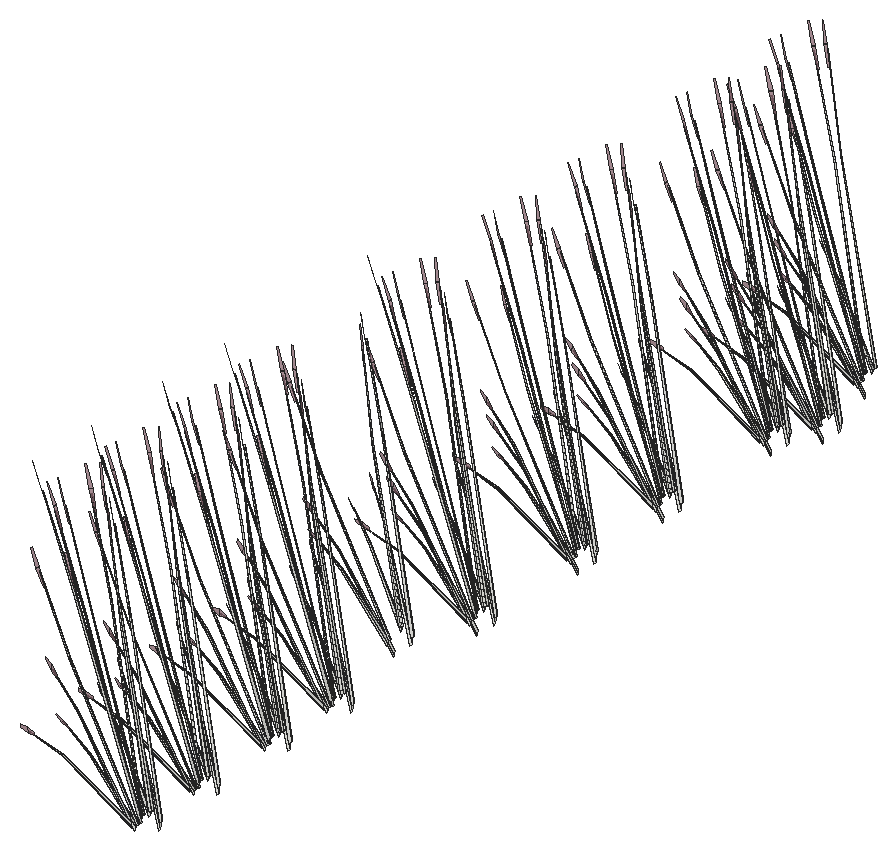
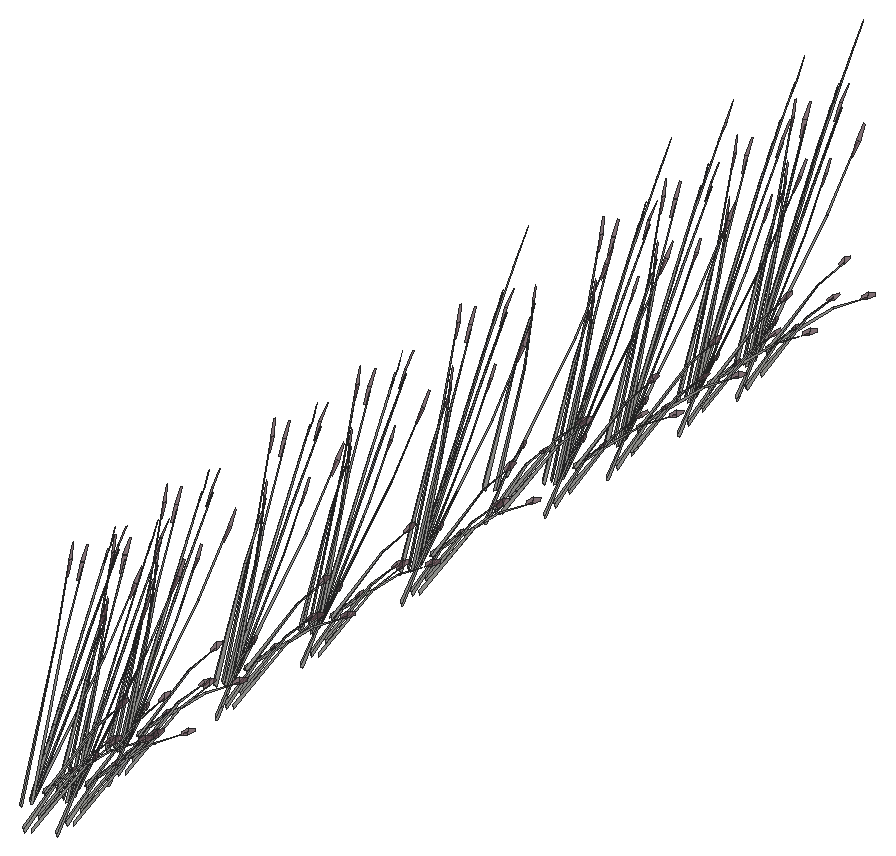
# SketchUp Ruby script. Lengths in inches.
U = 1.inch
M = Sketchup.active_model
def pt(a) = Geom::Point3d.new(a.map { |v| v * U })
def face(e, loops, mat)
  f = e.add_face(loops[0].map { |a| pt(a) })
  loops[1..].each { |l| e.add_face(l.map { |a| pt(a) }).erase! }
  f.material = f.back_material = mat if mat
  f
end
# faces: each face lists its corners as indices into pts; further lists are holes
def faces(e, pts, list, mat = nil) = list.each { |f| face(e, (f[0].is_a?(Array) ? f : [f]).map { |l| l.map { |i| pts[i] } }, mat) }
# xy, xz, yz: faces in a plane at the given z, y or x. An outline is a flat list of corners, or four numbers for a rectangle; further outlines are holes
def ring(l) = l.size == 4 ? [[l[0], l[1]], [l[2], l[1]], [l[2], l[3]], [l[0], l[3]]] : l.each_slice(2).to_a
def flat(e, list, mat, &to3) = list.each { |f| face(e, (f[0].is_a?(Array) ? f : [f]).map { |l| ring(l).map { |u, v| to3.(u, v) } }, mat) }
def xy(e, z, list, mat = nil) = flat(e, list, mat) { |x, y| [x, y, z] }
def xz(e, y, list, mat = nil) = flat(e, list, mat) { |x, z| [x, y, z] }
def yz(e, x, list, mat = nil) = flat(e, list, mat) { |y, z| [x, y, z] }
def lines(e, pts, list) = list.each { |a, b| e.add_line(pt(pts[a]), pt(pts[b])) }
# prism: a flat outline (further loops are holes) pulled along v
def prism(e, loops, v, mat = nil)
  f = face(e, loops, mat); d = Geom::Vector3d.new(v.map { |x| x * U })
  f.pushpull(f.normal.samedirection?(d) ? d.length : -d.length)
end
def box(e, o, s, mat = nil) = prism(e, [[o, [o[0] + s[0], o[1], o[2]], [o[0] + s[0], o[1] + s[1], o[2]], [o[0], o[1] + s[1], o[2]]]], [0, 0, s[2]], mat)
def at(x, y, z, deg = 0) = Geom::Transformation.translation(pt([x, y, z])) * Geom::Transformation.rotation(ORIGIN, Z_AXIS, deg.degrees)
def axes(o, x, y, z) = Geom::Transformation.new([*x, 0, *y, 0, *z, 0, *pt(o).to_a, 1])
def part(name) = M.definitions.add(name)
# library, detail: a bought-in or finely detailed component or shape, given as its bounding box
def library(name, o, s) = part(name).tap { |d| box(d.entities, o, s) }
def detail(e, o, s) = box(e.add_group.entities, o, s)
def put(e, d, t, mat = nil) = e.add_instance(d, t).tap { |i| i.material = mat if mat }
def group(e, t, mat = nil) = e.add_group.tap { |g| g.transformation = t; g.material = mat if mat }.entities
root = M.entities
M.materials.add("LightPink_Translucent").color = [144, 107, 117]
M.materials["LightPink_Translucent"].alpha = 0.75
c1 = part("blade")
p = [[2.15,0.21,22],[0,0.17,0],[0.09,0.45,0],[2.18,0.31,22],[2.29,0.31,22],[0.38,0.45,0],
  [2.48,0.24,33],[2.49,0.24,33],[2.48,0.22,33]]
faces(c1.entities,p,[[0,1,2,3],[4,5,2,3],[6,3,4,7],[8,0,3,6]])
c2 = part("seeds")
p = [[0.3,-0.1,1.38],[-0.01,-0.03,1.59],[-0.01,-0.03,0.03],[0.14,-0.07,-0.07],[0.29,-0.03,3],[0.15,0.01,3.11]]
faces(c2.entities,p,[[0,1,2,3],[1,0,4,5]],"LightPink_Translucent")
c3 = part("blade with seeds")
put(c3.entities,c1,at(0,0,0))
put(c3.entities,c2,axes([2.4,0.25,30.99],[1.5799,-0.05474,1.17369],[-0.12525,1.92788,0.29478],[-0.07173,-0.02425,1.56792]))
put(root,c3,axes([340.12,103.96,7.49],[0.02269,0.10283,1.76342],[-0.45738,0.53699,-0.26939],[-0.32488,-0.02707,0.30037]))
put(root,c3,axes([340.12,117.96,3.79],[0.02269,0.10283,1.76342],[-0.45738,0.53699,-0.26939],[-0.32488,-0.02707,0.30037]))
put(root,c3,axes([340.12,134.9,3.79],[0.02269,0.10283,1.76342],[-0.45738,0.53699,-0.26939],[-0.32488,-0.02707,0.30037]))
put(root,c3,axes([340.12,149.25,3.79],[0.02269,0.10283,1.76342],[-0.45738,0.53699,-0.26939],[-0.32488,-0.02707,0.30037]))
put(root,c3,axes([340.12,167.42,3.79],[0.02269,0.10283,1.76342],[-0.45738,0.53699,-0.26939],[-0.32488,-0.02707,0.30037]))
put(root,c3,axes([340.12,176.07,1.49],[0.02269,0.10283,1.76342],[-0.45738,0.53699,-0.26939],[-0.32488,-0.02707,0.30037]))
put(root,c3,axes([340.12,183.24,3.79],[0.02269,0.10283,1.76342],[-0.45738,0.53699,-0.26939],[-0.32488,-0.02707,0.30037]))
put(root,c3,axes([340.25,59.13,7],[0.06632,0.06511,1.77383],[-0.31973,0.58531,-0.16761],[-0.32381,0.00424,0.31391]))
put(root,c3,axes([340.25,68.96,7],[0.06632,0.06511,1.77383],[-0.31973,0.58531,-0.16761],[-0.32381,0.00424,0.31391]))
put(root,c3,axes([340.25,80.96,7],[0.06632,0.06511,1.77383],[-0.31973,0.58531,-0.16761],[-0.32381,0.00424,0.31391]))
put(root,c3,axes([340.25,91.43,7],[0.06632,0.06511,1.77383],[-0.31973,0.58531,-0.16761],[-0.32381,0.00424,0.31391]))
put(root,c3,axes([340.25,115.51,7],[0.06632,0.06511,1.77383],[-0.31973,0.58531,-0.16761],[-0.32381,0.00424,0.31391]))
put(root,c3,axes([340.25,132.45,7],[0.06632,0.06511,1.77383],[-0.31973,0.58531,-0.16761],[-0.32381,0.00424,0.31391]))
put(root,c3,axes([340.25,146.79,7],[0.06632,0.06511,1.77383],[-0.31973,0.58531,-0.16761],[-0.32381,0.00424,0.31391]))
put(root,c3,axes([340.25,164.96,7],[0.06632,0.06511,1.77383],[-0.31973,0.58531,-0.16761],[-0.32381,0.00424,0.31391]))
put(root,c3,axes([340.25,173.61,4.71],[0.06632,0.06511,1.77383],[-0.31973,0.58531,-0.16761],[-0.32381,0.00424,0.31391]))
put(root,c3,axes([340.25,180.78,7],[0.06632,0.06511,1.77383],[-0.31973,0.58531,-0.16761],[-0.32381,0.00424,0.31391]))
put(root,c3,axes([338.89,64.17,5.06],[0.37283,-0.29571,1.1486],[0.14711,0.46813,0.84392],[-0.26943,0.08382,0.25299]))
put(root,c3,axes([338.89,73.99,5.06],[0.37283,-0.29571,1.1486],[0.14711,0.46813,0.84392],[-0.26943,0.08382,0.25299]))
put(root,c3,axes([338.89,85.99,5.06],[0.37283,-0.29571,1.1486],[0.14711,0.46813,0.84392],[-0.26943,0.08382,0.25299]))
put(root,c3,axes([338.89,96.46,5.06],[0.37283,-0.29571,1.1486],[0.14711,0.46813,0.84392],[-0.26943,0.08382,0.25299]))
put(root,c3,axes([338.89,106.53,8.77],[0.37283,-0.29571,1.1486],[0.14711,0.46813,0.84392],[-0.26943,0.08382,0.25299]))
put(root,c3,axes([338.89,120.54,5.06],[0.37283,-0.29571,1.1486],[0.14711,0.46813,0.84392],[-0.26943,0.08382,0.25299]))
put(root,c3,axes([338.89,137.48,5.06],[0.37283,-0.29571,1.1486],[0.14711,0.46813,0.84392],[-0.26943,0.08382,0.25299]))
put(root,c3,axes([338.89,151.83,5.06],[0.37283,-0.29571,1.1486],[0.14711,0.46813,0.84392],[-0.26943,0.08382,0.25299]))
put(root,c3,axes([338.89,169.99,5.06],[0.37283,-0.29571,1.1486],[0.14711,0.46813,0.84392],[-0.26943,0.08382,0.25299]))
put(root,c3,axes([338.89,178.64,2.77],[0.37283,-0.29571,1.1486],[0.14711,0.46813,0.84392],[-0.26943,0.08382,0.25299]))
put(root,c3,axes([338.89,185.8125,5.06],[0.37283,-0.29571,1.1486],[0.14711,0.46813,0.84392],[-0.26943,0.08382,0.25299]))
put(root,c3,axes([340.99,58.74,7.01],[-0.19249,-0.00461,1.74944],[-0.61281,0.46055,-0.27667],[-0.32697,-0.0941,0.14031]))
put(root,c3,axes([340.99,68.57,7.01],[-0.19249,-0.00461,1.74944],[-0.61281,0.46055,-0.27667],[-0.32697,-0.0941,0.14031]))
put(root,c3,axes([340.99,80.57,7.01],[-0.19249,-0.00461,1.74944],[-0.61281,0.46055,-0.27667],[-0.32697,-0.0941,0.14031]))
put(root,c3,axes([340.99,91.04,7.01],[-0.19249,-0.00461,1.74944],[-0.61281,0.46055,-0.27667],[-0.32697,-0.0941,0.14031]))
put(root,c3,axes([340.99,115.12,7.01],[-0.19249,-0.00461,1.74944],[-0.61281,0.46055,-0.27667],[-0.32697,-0.0941,0.14031]))
put(root,c3,axes([340.99,132.06,7.01],[-0.19249,-0.00461,1.74944],[-0.61281,0.46055,-0.27667],[-0.32697,-0.0941,0.14031]))
put(root,c3,axes([340.99,146.4,7.01],[-0.19249,-0.00461,1.74944],[-0.61281,0.46055,-0.27667],[-0.32697,-0.0941,0.14031]))
put(root,c3,axes([340.99,164.57,7.01],[-0.19249,-0.00461,1.74944],[-0.61281,0.46055,-0.27667],[-0.32697,-0.0941,0.14031]))
put(root,c3,axes([340.99,173.22,4.72],[-0.19249,-0.00461,1.74944],[-0.61281,0.46055,-0.27667],[-0.32697,-0.0941,0.14031]))
put(root,c3,axes([340.99,180.39,7.01],[-0.19249,-0.00461,1.74944],[-0.61281,0.46055,-0.27667],[-0.32697,-0.0941,0.14031]))
put(root,c3,axes([340.2,61.29,7.03],[0.25275,-0.59491,0.48003],[0.83094,0.20343,0.3958],[-0.32677,0.03575,0.9933]))
put(root,c3,axes([340.2,71.12,7.03],[0.25275,-0.59491,0.48003],[0.83094,0.20343,0.3958],[-0.32677,0.03575,0.9933]))
put(root,c3,axes([340.2,83.12,7.03],[0.25275,-0.59491,0.48003],[0.83094,0.20343,0.3958],[-0.32677,0.03575,0.9933]))
put(root,c3,axes([340.2,93.59,7.03],[0.25275,-0.59491,0.48003],[0.83094,0.20343,0.3958],[-0.32677,0.03575,0.9933]))
put(root,c3,axes([340.2,117.66,7.03],[0.25275,-0.59491,0.48003],[0.83094,0.20343,0.3958],[-0.32677,0.03575,0.9933]))
put(root,c3,axes([340.2,134.6,7.03],[0.25275,-0.59491,0.48003],[0.83094,0.20343,0.3958],[-0.32677,0.03575,0.9933]))
put(root,c3,axes([340.2,148.95,7.03],[0.25275,-0.59491,0.48003],[0.83094,0.20343,0.3958],[-0.32677,0.03575,0.9933]))
put(root,c3,axes([340.2,167.12,7.03],[0.25275,-0.59491,0.48003],[0.83094,0.20343,0.3958],[-0.32677,0.03575,0.9933]))
put(root,c3,axes([340.2,175.77,4.73],[0.25275,-0.59491,0.48003],[0.83094,0.20343,0.3958],[-0.32677,0.03575,0.9933]))
put(root,c3,axes([340.2,182.9375,7.03],[0.25275,-0.59491,0.48003],[0.83094,0.20343,0.3958],[-0.32677,0.03575,0.9933]))
put(root,c3,axes([340.5,61.12,7.33],[0.45012,0.59081,-0.1216],[-0.79888,0.29033,-0.67495],[-0.33665,0.07795,1.02557]))
put(root,c3,axes([340.5,70.95,7.33],[0.45012,0.59081,-0.1216],[-0.79888,0.29033,-0.67495],[-0.33665,0.07795,1.02557]))
put(root,c3,axes([340.5,82.95,7.33],[0.45012,0.59081,-0.1216],[-0.79888,0.29033,-0.67495],[-0.33665,0.07795,1.02557]))
put(root,c3,axes([340.5,93.42,7.33],[0.45012,0.59081,-0.1216],[-0.79888,0.29033,-0.67495],[-0.33665,0.07795,1.02557]))
put(root,c3,axes([340.5,117.49,7.33],[0.45012,0.59081,-0.1216],[-0.79888,0.29033,-0.67495],[-0.33665,0.07795,1.02557]))
put(root,c3,axes([340.5,134.43,7.33],[0.45012,0.59081,-0.1216],[-0.79888,0.29033,-0.67495],[-0.33665,0.07795,1.02557]))
put(root,c3,axes([340.5,148.78,7.33],[0.45012,0.59081,-0.1216],[-0.79888,0.29033,-0.67495],[-0.33665,0.07795,1.02557]))
put(root,c3,axes([340.5,166.94,7.33],[0.45012,0.59081,-0.1216],[-0.79888,0.29033,-0.67495],[-0.33665,0.07795,1.02557]))
put(root,c3,axes([340.5,175.6,5.03],[0.45012,0.59081,-0.1216],[-0.79888,0.29033,-0.67495],[-0.33665,0.07795,1.02557]))
put(root,c3,axes([340.5,182.77,7.33],[0.45012,0.59081,-0.1216],[-0.79888,0.29033,-0.67495],[-0.33665,0.07795,1.02557]))
put(root,c3,axes([341.51,59.89,7.33],[-0.0479,0.66354,-0.1216],[-0.90696,-0.01814,-0.67495],[-0.3493,-0.04609,1.02557]))
put(root,c3,axes([341.51,69.72,7.33],[-0.0479,0.66354,-0.1216],[-0.90696,-0.01814,-0.67495],[-0.3493,-0.04609,1.02557]))
put(root,c3,axes([341.51,81.72,7.33],[-0.0479,0.66354,-0.1216],[-0.90696,-0.01814,-0.67495],[-0.3493,-0.04609,1.02557]))
put(root,c3,axes([341.51,92.19,7.33],[-0.0479,0.66354,-0.1216],[-0.90696,-0.01814,-0.67495],[-0.3493,-0.04609,1.02557]))
put(root,c3,axes([341.51,116.27,7.33],[-0.0479,0.66354,-0.1216],[-0.90696,-0.01814,-0.67495],[-0.3493,-0.04609,1.02557]))
put(root,c3,axes([341.51,133.21,7.33],[-0.0479,0.66354,-0.1216],[-0.90696,-0.01814,-0.67495],[-0.3493,-0.04609,1.02557]))
put(root,c3,axes([341.51,147.55,7.33],[-0.0479,0.66354,-0.1216],[-0.90696,-0.01814,-0.67495],[-0.3493,-0.04609,1.02557]))
put(root,c3,axes([341.51,165.72,7.33],[-0.0479,0.66354,-0.1216],[-0.90696,-0.01814,-0.67495],[-0.3493,-0.04609,1.02557]))
put(root,c3,axes([341.51,174.37,5.03],[-0.0479,0.66354,-0.1216],[-0.90696,-0.01814,-0.67495],[-0.3493,-0.04609,1.02557]))
put(root,c3,axes([341.51,181.54,7.33],[-0.0479,0.66354,-0.1216],[-0.90696,-0.01814,-0.67495],[-0.3493,-0.04609,1.02557]))
put(root,c3,axes([340.92,59.9375,6.82],[-0.50902,-0.40851,-0.35414],[0.58122,-0.38671,0.4572],[-0.29531,-0.05884,0.87481]))
put(root,c3,axes([340.92,69.77,6.82],[-0.50902,-0.40851,-0.35414],[0.58122,-0.38671,0.4572],[-0.29531,-0.05884,0.87481]))
put(root,c3,axes([340.92,81.77,6.82],[-0.50902,-0.40851,-0.35414],[0.58122,-0.38671,0.4572],[-0.29531,-0.05884,0.87481]))
put(root,c3,axes([340.92,92.24,6.82],[-0.50902,-0.40851,-0.35414],[0.58122,-0.38671,0.4572],[-0.29531,-0.05884,0.87481]))
put(root,c3,axes([340.92,102.3,10.53],[-0.50902,-0.40851,-0.35414],[0.58122,-0.38671,0.4572],[-0.29531,-0.05884,0.87481]))
put(root,c3,axes([340.92,116.3125,6.82],[-0.50902,-0.40851,-0.35414],[0.58122,-0.38671,0.4572],[-0.29531,-0.05884,0.87481]))
put(root,c3,axes([340.92,133.25,6.82],[-0.50902,-0.40851,-0.35414],[0.58122,-0.38671,0.4572],[-0.29531,-0.05884,0.87481]))
put(root,c3,axes([340.92,147.6,6.82],[-0.50902,-0.40851,-0.35414],[0.58122,-0.38671,0.4572],[-0.29531,-0.05884,0.87481]))
put(root,c3,axes([340.92,165.76,6.82],[-0.50902,-0.40851,-0.35414],[0.58122,-0.38671,0.4572],[-0.29531,-0.05884,0.87481]))
put(root,c3,axes([340.92,174.42,4.53],[-0.50902,-0.40851,-0.35414],[0.58122,-0.38671,0.4572],[-0.29531,-0.05884,0.87481]))
put(root,c3,axes([340.92,181.59,6.82],[-0.50902,-0.40851,-0.35414],[0.58122,-0.38671,0.4572],[-0.29531,-0.05884,0.87481]))
put(root,c3,axes([340.14,61.13,7.02],[-0.32857,-0.44488,0.0643],[0.59916,-0.21775,0.50621],[-0.26412,0.04296,0.77189]))
put(root,c3,axes([340.14,70.96,7.02],[-0.32857,-0.44488,0.0643],[0.59916,-0.21775,0.50621],[-0.26412,0.04296,0.77189]))
put(root,c3,axes([340.14,82.96,7.02],[-0.32857,-0.44488,0.0643],[0.59916,-0.21775,0.50621],[-0.26412,0.04296,0.77189]))
put(root,c3,axes([340.14,93.43,7.02],[-0.32857,-0.44488,0.0643],[0.59916,-0.21775,0.50621],[-0.26412,0.04296,0.77189]))
put(root,c3,axes([340.14,117.51,7.02],[-0.32857,-0.44488,0.0643],[0.59916,-0.21775,0.50621],[-0.26412,0.04296,0.77189]))
put(root,c3,axes([340.14,134.45,7.02],[-0.32857,-0.44488,0.0643],[0.59916,-0.21775,0.50621],[-0.26412,0.04296,0.77189]))
put(root,c3,axes([340.14,148.79,7.02],[-0.32857,-0.44488,0.0643],[0.59916,-0.21775,0.50621],[-0.26412,0.04296,0.77189]))
put(root,c3,axes([340.14,166.96,7.02],[-0.32857,-0.44488,0.0643],[0.59916,-0.21775,0.50621],[-0.26412,0.04296,0.77189]))
put(root,c3,axes([340.14,175.61,4.73],[-0.32857,-0.44488,0.0643],[0.59916,-0.21775,0.50621],[-0.26412,0.04296,0.77189]))
put(root,c3,axes([340.14,182.78,7.02],[-0.32857,-0.44488,0.0643],[0.59916,-0.21775,0.50621],[-0.26412,0.04296,0.77189]))
put(root,c3,axes([341.64,62.36,6.17],[0.22344,-0.20048,1.71376],[0.56419,0.54113,0.13857],[-0.38697,0.24643,0.73262]))
put(root,c3,axes([341.64,72.19,6.17],[0.22344,-0.20048,1.71376],[0.56419,0.54113,0.13857],[-0.38697,0.24643,0.73262]))
put(root,c3,axes([341.64,84.19,6.17],[0.22344,-0.20048,1.71376],[0.56419,0.54113,0.13857],[-0.38697,0.24643,0.73262]))
put(root,c3,axes([341.64,94.66,6.17],[0.22344,-0.20048,1.71376],[0.56419,0.54113,0.13857],[-0.38697,0.24643,0.73262]))
put(root,c3,axes([341.64,104.73,9.875],[0.22344,-0.20048,1.71376],[0.56419,0.54113,0.13857],[-0.38697,0.24643,0.73262]))
put(root,c3,axes([341.64,118.74,6.17],[0.22344,-0.20048,1.71376],[0.56419,0.54113,0.13857],[-0.38697,0.24643,0.73262]))
put(root,c3,axes([341.64,135.68,6.17],[0.22344,-0.20048,1.71376],[0.56419,0.54113,0.13857],[-0.38697,0.24643,0.73262]))
put(root,c3,axes([341.64,150.02,6.17],[0.22344,-0.20048,1.71376],[0.56419,0.54113,0.13857],[-0.38697,0.24643,0.73262]))
put(root,c3,axes([341.64,168.1875,6.17],[0.22344,-0.20048,1.71376],[0.56419,0.54113,0.13857],[-0.38697,0.24643,0.73262]))
put(root,c3,axes([341.64,176.84,3.875],[0.22344,-0.20048,1.71376],[0.56419,0.54113,0.13857],[-0.38697,0.24643,0.73262]))
put(root,c3,axes([340.3,62.89,6.82],[-0.77872,0.09325,-0.35414],[-0.20563,-0.53305,0.4572],[-0.22316,0.14318,0.87481]))
put(root,c3,axes([340.3,72.71,6.82],[-0.77872,0.09325,-0.35414],[-0.20563,-0.53305,0.4572],[-0.22316,0.14318,0.87481]))
put(root,c3,axes([340.3,84.71,6.82],[-0.77872,0.09325,-0.35414],[-0.20563,-0.53305,0.4572],[-0.22316,0.14318,0.87481]))
put(root,c3,axes([340.3,95.19,6.82],[-0.77872,0.09325,-0.35414],[-0.20563,-0.53305,0.4572],[-0.22316,0.14318,0.87481]))
put(root,c3,axes([340.3,105.25,10.53],[-0.77872,0.09325,-0.35414],[-0.20563,-0.53305,0.4572],[-0.22316,0.14318,0.87481]))
put(root,c3,axes([340.3,119.26,6.82],[-0.77872,0.09325,-0.35414],[-0.20563,-0.53305,0.4572],[-0.22316,0.14318,0.87481]))
put(root,c3,axes([340.3,136.2,6.82],[-0.77872,0.09325,-0.35414],[-0.20563,-0.53305,0.4572],[-0.22316,0.14318,0.87481]))
put(root,c3,axes([340.3,150.55,6.82],[-0.77872,0.09325,-0.35414],[-0.20563,-0.53305,0.4572],[-0.22316,0.14318,0.87481]))
put(root,c3,axes([340.3,168.71,6.82],[-0.77872,0.09325,-0.35414],[-0.20563,-0.53305,0.4572],[-0.22316,0.14318,0.87481]))
put(root,c3,axes([340.3,177.37,4.53],[-0.77872,0.09325,-0.35414],[-0.20563,-0.53305,0.4572],[-0.22316,0.14318,0.87481]))
put(root,c3,axes([339.875,64.47,3.79],[0.12,0.06519,1.76342],[0.20347,0.60397,-0.26939],[-0.26596,0.12879,0.30037]))
put(root,c3,axes([339.875,74.3,3.79],[0.12,0.06519,1.76342],[0.20347,0.60397,-0.26939],[-0.26596,0.12879,0.30037]))
put(root,c3,axes([339.875,86.3,3.79],[0.12,0.06519,1.76342],[0.20347,0.60397,-0.26939],[-0.26596,0.12879,0.30037]))
put(root,c3,axes([339.875,96.77,3.79],[0.12,0.06519,1.76342],[0.20347,0.60397,-0.26939],[-0.26596,0.12879,0.30037]))
put(root,c3,axes([339.875,106.84,7.49],[0.12,0.06519,1.76342],[0.20347,0.60397,-0.26939],[-0.26596,0.12879,0.30037]))
put(root,c3,axes([339.875,120.84,3.79],[0.12,0.06519,1.76342],[0.20347,0.60397,-0.26939],[-0.26596,0.12879,0.30037]))
put(root,c3,axes([339.875,137.78,3.79],[0.12,0.06519,1.76342],[0.20347,0.60397,-0.26939],[-0.26596,0.12879,0.30037]))
put(root,c3,axes([339.875,152.13,3.79],[0.12,0.06519,1.76342],[0.20347,0.60397,-0.26939],[-0.26596,0.12879,0.30037]))
put(root,c3,axes([339.875,170.3,3.79],[0.12,0.06519,1.76342],[0.20347,0.60397,-0.26939],[-0.26596,0.12879,0.30037]))
put(root,c3,axes([339.875,178.95,1.49],[0.12,0.06519,1.76342],[0.20347,0.60397,-0.26939],[-0.26596,0.12879,0.30037]))
put(root,c3,axes([339.7,60.92,5.06],[0.57115,-0.04669,1.1486],[-0.36229,0.41137,0.84392],[-0.28224,-0.06171,0.25299]))
put(root,c3,axes([339.7,70.74,5.06],[0.57115,-0.04669,1.1486],[-0.36229,0.41137,0.84392],[-0.28224,-0.06171,0.25299]))
put(root,c3,axes([339.7,82.74,5.06],[0.57115,-0.04669,1.1486],[-0.36229,0.41137,0.84392],[-0.28224,-0.06171,0.25299]))
put(root,c3,axes([339.7,93.22,5.06],[0.57115,-0.04669,1.1486],[-0.36229,0.41137,0.84392],[-0.28224,-0.06171,0.25299]))
put(root,c3,axes([339.7,103.28,8.77],[0.57115,-0.04669,1.1486],[-0.36229,0.41137,0.84392],[-0.28224,-0.06171,0.25299]))
put(root,c3,axes([339.7,117.29,5.06],[0.57115,-0.04669,1.1486],[-0.36229,0.41137,0.84392],[-0.28224,-0.06171,0.25299]))
put(root,c3,axes([339.7,134.23,5.06],[0.57115,-0.04669,1.1486],[-0.36229,0.41137,0.84392],[-0.28224,-0.06171,0.25299]))
put(root,c3,axes([339.7,148.58,5.06],[0.57115,-0.04669,1.1486],[-0.36229,0.41137,0.84392],[-0.28224,-0.06171,0.25299]))
put(root,c3,axes([339.7,166.74,5.06],[0.57115,-0.04669,1.1486],[-0.36229,0.41137,0.84392],[-0.28224,-0.06171,0.25299]))
put(root,c3,axes([339.7,175.4,2.77],[0.57115,-0.04669,1.1486],[-0.36229,0.41137,0.84392],[-0.28224,-0.06171,0.25299]))
put(root,c3,axes([339.7,182.56,5.06],[0.57115,-0.04669,1.1486],[-0.36229,0.41137,0.84392],[-0.28224,-0.06171,0.25299]))
put(root,c3,axes([340.4,62.77,7.03],[-0.22187,-0.60049,0.48003],[0.87033,-0.10422,0.3958],[-0.25651,0.14123,0.9933]))
put(root,c3,axes([340.4,72.6,7.03],[-0.22187,-0.60049,0.48003],[0.87033,-0.10422,0.3958],[-0.25651,0.14123,0.9933]))
put(root,c3,axes([340.4,84.6,7.03],[-0.22187,-0.60049,0.48003],[0.87033,-0.10422,0.3958],[-0.25651,0.14123,0.9933]))
put(root,c3,axes([340.4,95.07,7.03],[-0.22187,-0.60049,0.48003],[0.87033,-0.10422,0.3958],[-0.25651,0.14123,0.9933]))
put(root,c3,axes([340.4,119.15,7.03],[-0.22187,-0.60049,0.48003],[0.87033,-0.10422,0.3958],[-0.25651,0.14123,0.9933]))
put(root,c3,axes([340.4,136.09,7.03],[-0.22187,-0.60049,0.48003],[0.87033,-0.10422,0.3958],[-0.25651,0.14123,0.9933]))
put(root,c3,axes([340.4,150.43,7.03],[-0.22187,-0.60049,0.48003],[0.87033,-0.10422,0.3958],[-0.25651,0.14123,0.9933]))
put(root,c3,axes([340.4,168.6,7.03],[-0.22187,-0.60049,0.48003],[0.87033,-0.10422,0.3958],[-0.25651,0.14123,0.9933]))
put(root,c3,axes([340.4,177.25,4.73],[-0.22187,-0.60049,0.48003],[0.87033,-0.10422,0.3958],[-0.25651,0.14123,0.9933]))
put(root,c3,axes([340.4,184.42,7.03],[-0.22187,-0.60049,0.48003],[0.87033,-0.10422,0.3958],[-0.25651,0.14123,0.9933]))
put(root,c3,axes([340.85,59.79,7.39],[0.7388,-0.48151,0.53763],[0.63717,0.51135,0.4433],[-0.34662,-0.08882,1.11249]))
put(root,c3,axes([340.85,69.61,7.39],[0.7388,-0.48151,0.53763],[0.63717,0.51135,0.4433],[-0.34662,-0.08882,1.11249]))
put(root,c3,axes([340.85,81.61,7.39],[0.7388,-0.48151,0.53763],[0.63717,0.51135,0.4433],[-0.34662,-0.08882,1.11249]))
put(root,c3,axes([340.85,92.08,7.39],[0.7388,-0.48151,0.53763],[0.63717,0.51135,0.4433],[-0.34662,-0.08882,1.11249]))
put(root,c3,axes([340.85,116.16,7.39],[0.7388,-0.48151,0.53763],[0.63717,0.51135,0.4433],[-0.34662,-0.08882,1.11249]))
